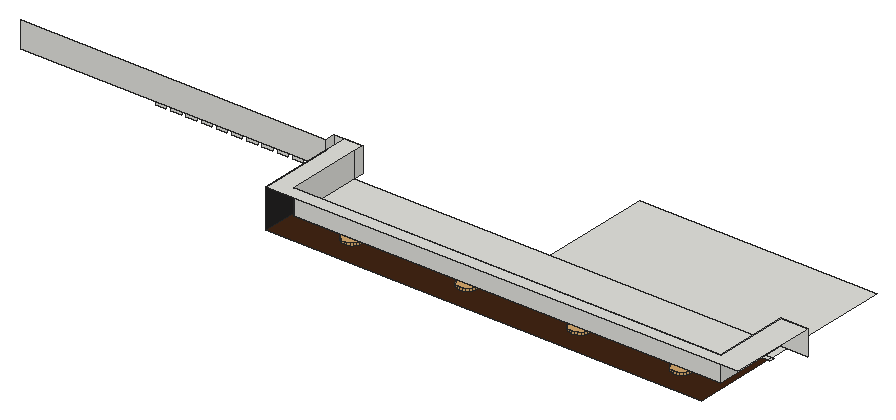
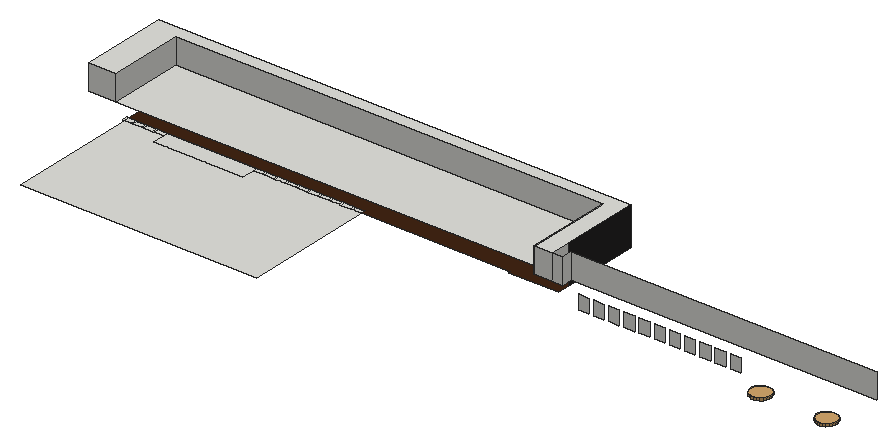
# SketchUp Ruby script. Lengths in inches.
U = 1.inch
M = Sketchup.active_model
def pt(a) = Geom::Point3d.new(a.map { |v| v * U })
def face(e, loops, mat)
  f = e.add_face(loops[0].map { |a| pt(a) })
  loops[1..].each { |l| e.add_face(l.map { |a| pt(a) }).erase! }
  f.material = f.back_material = mat if mat
  f
end
# faces: each face lists its corners as indices into pts; further lists are holes
def faces(e, pts, list, mat = nil) = list.each { |f| face(e, (f[0].is_a?(Array) ? f : [f]).map { |l| l.map { |i| pts[i] } }, mat) }
# xy, xz, yz: faces in a plane at the given z, y or x. An outline is a flat list of corners, or four numbers for a rectangle; further outlines are holes
def ring(l) = l.size == 4 ? [[l[0], l[1]], [l[2], l[1]], [l[2], l[3]], [l[0], l[3]]] : l.each_slice(2).to_a
def flat(e, list, mat, &to3) = list.each { |f| face(e, (f[0].is_a?(Array) ? f : [f]).map { |l| ring(l).map { |u, v| to3.(u, v) } }, mat) }
def xy(e, z, list, mat = nil) = flat(e, list, mat) { |x, y| [x, y, z] }
def xz(e, y, list, mat = nil) = flat(e, list, mat) { |x, z| [x, y, z] }
def yz(e, x, list, mat = nil) = flat(e, list, mat) { |y, z| [x, y, z] }
def lines(e, pts, list) = list.each { |a, b| e.add_line(pt(pts[a]), pt(pts[b])) }
# prism: a flat outline (further loops are holes) pulled along v
def prism(e, loops, v, mat = nil)
  f = face(e, loops, mat); d = Geom::Vector3d.new(v.map { |x| x * U })
  f.pushpull(f.normal.samedirection?(d) ? d.length : -d.length)
end
def box(e, o, s, mat = nil) = prism(e, [[o, [o[0] + s[0], o[1], o[2]], [o[0] + s[0], o[1] + s[1], o[2]], [o[0], o[1] + s[1], o[2]]]], [0, 0, s[2]], mat)
def at(x, y, z, deg = 0) = Geom::Transformation.translation(pt([x, y, z])) * Geom::Transformation.rotation(ORIGIN, Z_AXIS, deg.degrees)
def axes(o, x, y, z) = Geom::Transformation.new([*x, 0, *y, 0, *z, 0, *pt(o).to_a, 1])
def part(name) = M.definitions.add(name)
# library, detail: a bought-in or finely detailed component or shape, given as its bounding box
def library(name, o, s) = part(name).tap { |d| box(d.entities, o, s) }
def detail(e, o, s) = box(e.add_group.entities, o, s)
def put(e, d, t, mat = nil) = e.add_instance(d, t).tap { |i| i.material = mat if mat }
def group(e, t, mat = nil) = e.add_group.tap { |g| g.transformation = t; g.material = mat if mat }.entities
root = M.entities
M.materials.add("[Field Square Tile]").color = [211, 167, 108]
M.materials.add("[Granite Dark Gray]").color = [38, 37, 37]
M.materials.add("[Wood Veneer 01]").color = [66, 38, 20]
xy(root,380.5,[[534.46,2343.96,539.88,2346.71],[539.88,2343.96,541.08,2346.71],[541.08,2343.96,546.51,2346.71],[546.51,2343.96,547.71,2346.71],[547.71,2343.96,553.13,2346.71],
  [553.13,2343.96,554.33,2346.71],[554.33,2343.96,559.76,2346.71],[559.76,2343.96,560.96,2346.71],[560.96,2343.96,566.38,2346.71],[566.38,2343.96,567.58,2346.71],
  [567.58,2343.96,573.01,2346.71],[573.01,2343.96,574.21,2346.71],[574.21,2343.96,579.63,2346.71],[579.63,2343.96,580.83,2346.71],[580.83,2343.96,586.26,2346.71],
  [586.26,2343.96,587.46,2346.71],[587.46,2343.96,592.88,2346.71],[592.88,2343.96,594.08,2346.71],[594.08,2343.96,599.51,2346.71],[599.51,2343.96,653.06,2354.27],
  [653.06,2343.96,658.48,2346.71],[658.48,2343.96,659.68,2346.71],[659.68,2343.96,665.11,2346.71],[665.11,2343.96,666.31,2346.71],[666.31,2343.96,671.73,2346.71],
  [671.73,2343.96,672.56,2346.71],[672.56,2343.96,676.54,2346.71],[676.54,2343.96,677.98,2346.71],[534.46,2346.71,534.46,2425.46,676.54,2425.46,676.54,2346.71,653.06,2346.71,653.06,2354.27,599.51,2354.27,599.51,2346.71]])
xy(root,380.5,[[[414.98,2294.125,414.98,2347.9,444.78,2347.9,444.78,2346.71,534.46,2346.71,534.46,2343.96,676.54,2343.96,676.54,2294.125],[521.68,2306.32,523.23,2306.53,524.68,2307.13,525.92,2308.08,526.88,2309.32,527.48,2310.77,527.68,2312.32,527.48,2313.88,526.88,2315.32,525.92,2316.57,524.68,2317.52,523.23,2318.12,521.68,2318.32,520.13,2318.12,518.68,2317.52,517.4375,2316.57,516.49,2315.32,515.89,2313.88,515.68,2312.32,515.89,2310.77,516.49,2309.32,517.4375,2308.08,518.68,2307.13,520.13,2306.53],[588.96,2306.32,590.51,2306.53,591.96,2307.13,593.2,2308.08,594.16,2309.32,594.76,2310.77,594.96,2312.32,594.76,2313.88,594.16,2315.32,593.2,2316.57,591.96,2317.52,590.51,2318.12,588.96,2318.32,587.41,2318.12,585.96,2317.52,584.72,2316.57,583.76,2315.32,583.16,2313.88,582.96,2312.32,583.16,2310.77,583.76,2309.32,584.72,2308.08,585.96,2307.13,587.41,2306.53],[650.33,2306.32,651.89,2306.53,653.33,2307.13,654.58,2308.08,655.53,2309.32,656.13,2310.77,656.33,2312.32,656.13,2313.88,655.53,2315.32,654.58,2316.57,653.33,2317.52,651.89,2318.12,650.33,2318.32,648.78,2318.12,647.33,2317.52,646.09,2316.57,645.14,2315.32,644.54,2313.88,644.33,2312.32,644.54,2310.77,645.14,2309.32,646.09,2308.08,647.33,2307.13,648.78,2306.53],[452.22,2306.32,453.77,2306.53,455.22,2307.13,456.46,2308.08,457.41,2309.32,458.01,2310.77,458.22,2312.32,458.01,2313.88,457.41,2315.32,456.46,2316.57,455.22,2317.52,453.77,2318.12,452.22,2318.32,450.67,2318.12,449.22,2317.52,447.98,2316.57,447.02,2315.32,446.42,2313.88,446.22,2312.32,446.42,2310.77,447.02,2309.32,447.98,2308.08,449.22,2307.13,450.67,2306.53]]],"[Wood Veneer 01]")
xy(root,381.8125,[[452.22,2306.32,450.67,2306.53,449.22,2307.13,447.98,2308.08,447.02,2309.32,446.42,2310.77,446.22,2312.32,446.42,2313.88,447.02,2315.32,447.98,2316.57,449.22,2317.52,450.67,2318.12,452.22,2318.32,453.77,2318.12,455.22,2317.52,456.46,2316.57,457.41,2315.32,458.01,2313.88,458.22,2312.32,458.01,2310.77,457.41,2309.32,456.46,2308.08,455.22,2307.13,453.77,2306.53],[521.68,2306.32,520.13,2306.53,518.68,2307.13,517.4375,2308.08,516.49,2309.32,515.89,2310.77,515.68,2312.32,515.89,2313.88,516.49,2315.32,517.4375,2316.57,518.68,2317.52,520.13,2318.12,521.68,2318.32,523.23,2318.12,524.68,2317.52,525.92,2316.57,526.88,2315.32,527.48,2313.88,527.68,2312.32,527.48,2310.77,526.88,2309.32,525.92,2308.08,524.68,2307.13,523.23,2306.53],[588.96,2306.32,587.41,2306.53,585.96,2307.13,584.72,2308.08,583.76,2309.32,583.16,2310.77,582.96,2312.32,583.16,2313.88,583.76,2315.32,584.72,2316.57,585.96,2317.52,587.41,2318.12,588.96,2318.32,590.51,2318.12,591.96,2317.52,593.2,2316.57,594.16,2315.32,594.76,2313.88,594.96,2312.32,594.76,2310.77,594.16,2309.32,593.2,2308.08,591.96,2307.13,590.51,2306.53],[650.33,2306.32,648.78,2306.53,647.33,2307.13,646.09,2308.08,645.14,2309.32,644.54,2310.77,644.33,2312.32,644.54,2313.88,645.14,2315.32,646.09,2316.57,647.33,2317.52,648.78,2318.12,650.33,2318.32,651.89,2318.12,653.33,2317.52,654.58,2316.57,655.53,2315.32,656.13,2313.88,656.33,2312.32,656.13,2310.77,655.53,2309.32,654.58,2308.08,653.33,2307.13,651.89,2306.53]],"[Field Square Tile]")
xy(root,381.875,[[240.83,2359.13,239.27,2359.16,237.76,2359.6,236.42,2360.41,235.34,2361.54,234.58,2362.91,234.21,2364.4375,234.24,2366,234.68,2367.51,235.49,2368.85,236.62,2369.93,237.99,2370.69,239.51,2371.06,241.08,2371.03,242.58,2370.59,243.92,2369.78,245.01,2368.65,245.76,2367.28,246.14,2365.75,246.1,2364.1875,245.67,2362.68,244.86,2361.34,243.73,2360.26,242.35,2359.51],[280.58,2359.13,279.02,2359.16,277.51,2359.6,276.17,2360.41,275.09,2361.54,274.33,2362.91,273.96,2364.4375,273.99,2366,274.43,2367.51,275.24,2368.85,276.37,2369.93,277.74,2370.69,279.26,2371.06,280.83,2371.03,282.33,2370.59,283.67,2369.78,284.76,2368.65,285.51,2367.28,285.89,2365.75,285.85,2364.1875,285.42,2362.68,284.61,2361.34,283.48,2360.26,282.1,2359.51]],"[Field Square Tile]")
xy(root,388.625,[[425.6875,2301.68,682.18,2346.71]])
xy(root,403.8125,[[414.98,2294.125,698.16,2294.125,698.16,2346.71,682.18,2346.71,682.18,2301.68,425.6875,2301.68,425.6875,2353.05,414.98,2353.05]])
xz(root,2301.68,[[425.6875,388.625,682.18,403.8125]])
xz(root,2346.49,[[225.31,388.625,408.63,403.8125]])
xz(root,2346.71,[[682.18,388.625,698.16,403.8125]])
xz(root,2353.05,[[408.63,388.625,414.98,403.8125],[414.98,388.625,425.6875,403.8125]])
xz(root,2355.06,[[299.93,380.5,306.18,388.625],[309.06,380.5,315.31,388.625],[318.18,380.5,324.43,388.625],[327.31,380.5,333.56,388.625],[336.43,380.5,342.68,388.625],
  [345.56,380.5,351.81,388.625],[354.68,380.5,360.93,388.625],[363.81,380.5,370.06,388.625],[372.93,380.5,379.18,388.625],[382.06,380.5,388.31,388.625],
  [391.18,380.5,397.43,388.625]])
yz(root,408.63,[[2346.49,388.625,2353.05,403.8125]])
yz(root,414.98,[[2294.125,380.5,2340.15,403.8125]],"[Granite Dark Gray]")
yz(root,425.6875,[[2301.68,388.625,2346.71,403.8125],[2346.71,388.625,2353.05,403.8125]])
yz(root,682.18,[[2301.68,388.625,2346.71,403.8125]])
p = [[452.22,2306.32,380.5],[450.67,2306.53,380.5],[450.67,2306.53,381.8125],[452.22,2306.32,381.8125],[453.77,2306.53,380.5],[453.77,2306.53,381.8125],
  [521.68,2306.32,380.5],[520.13,2306.53,380.5],[520.13,2306.53,381.8125],[521.68,2306.32,381.8125],[523.23,2306.53,380.5],[523.23,2306.53,381.8125],
  [588.96,2306.32,380.5],[587.41,2306.53,380.5],[587.41,2306.53,381.8125],[588.96,2306.32,381.8125],[590.51,2306.53,380.5],[590.51,2306.53,381.8125],
  [650.33,2306.32,380.5],[648.78,2306.53,380.5],[648.78,2306.53,381.8125],[650.33,2306.32,381.8125],[651.89,2306.53,380.5],[651.89,2306.53,381.8125],
  [449.22,2307.13,380.5],[449.22,2307.13,381.8125],[455.22,2307.13,380.5],[455.22,2307.13,381.8125],[518.68,2307.13,380.5],[518.68,2307.13,381.8125],
  [524.68,2307.13,380.5],[524.68,2307.13,381.8125],[585.96,2307.13,380.5],[585.96,2307.13,381.8125],[591.96,2307.13,380.5],[591.96,2307.13,381.8125],
  [647.33,2307.13,380.5],[647.33,2307.13,381.8125],[653.33,2307.13,380.5],[653.33,2307.13,381.8125],[447.98,2308.08,380.5],[447.98,2308.08,381.8125],
  [456.46,2308.08,380.5],[456.46,2308.08,381.8125],[517.4375,2308.08,380.5],[517.4375,2308.08,381.8125],[525.92,2308.08,380.5],[525.92,2308.08,381.8125],
  [584.72,2308.08,380.5],[584.72,2308.08,381.8125],[593.2,2308.08,380.5],[593.2,2308.08,381.8125],[646.09,2308.08,380.5],[646.09,2308.08,381.8125],
  [654.58,2308.08,380.5],[654.58,2308.08,381.8125],[447.02,2309.32,380.5],[447.02,2309.32,381.8125],[457.41,2309.32,380.5],[457.41,2309.32,381.8125],
  [516.49,2309.32,380.5],[516.49,2309.32,381.8125],[526.88,2309.32,380.5],[526.88,2309.32,381.8125],[583.76,2309.32,380.5],[583.76,2309.32,381.8125],
  [594.16,2309.32,380.5],[594.16,2309.32,381.8125],[645.14,2309.32,380.5],[645.14,2309.32,381.8125],[655.53,2309.32,380.5],[655.53,2309.32,381.8125],
  [446.42,2310.77,380.5],[446.42,2310.77,381.8125],[458.01,2310.77,380.5],[458.01,2310.77,381.8125],[515.89,2310.77,380.5],[515.89,2310.77,381.8125],
  [527.48,2310.77,380.5],[527.48,2310.77,381.8125],[583.16,2310.77,380.5],[583.16,2310.77,381.8125],[594.76,2310.77,380.5],[594.76,2310.77,381.8125],
  [644.54,2310.77,380.5],[644.54,2310.77,381.8125],[656.13,2310.77,380.5],[656.13,2310.77,381.8125],[446.22,2312.32,380.5],[446.22,2312.32,381.8125],
  [458.22,2312.32,380.5],[458.22,2312.32,381.8125],[515.68,2312.32,380.5],[515.68,2312.32,381.8125],[527.68,2312.32,380.5],[527.68,2312.32,381.8125],
  [582.96,2312.32,380.5],[582.96,2312.32,381.8125],[594.96,2312.32,380.5],[594.96,2312.32,381.8125],[644.33,2312.32,380.5],[644.33,2312.32,381.8125],
  [656.33,2312.32,380.5],[656.33,2312.32,381.8125],[446.42,2313.88,380.5],[446.42,2313.88,381.8125],[458.01,2313.88,380.5],[458.01,2313.88,381.8125],
  [515.89,2313.88,380.5],[515.89,2313.88,381.8125],[527.48,2313.88,380.5],[527.48,2313.88,381.8125],[583.16,2313.88,380.5],[583.16,2313.88,381.8125],
  [594.76,2313.88,380.5],[594.76,2313.88,381.8125],[644.54,2313.88,380.5],[644.54,2313.88,381.8125],[656.13,2313.88,380.5],[656.13,2313.88,381.8125],
  [447.02,2315.32,380.5],[447.02,2315.32,381.8125],[457.41,2315.32,380.5],[457.41,2315.32,381.8125],[516.49,2315.32,380.5],[516.49,2315.32,381.8125],
  [526.88,2315.32,380.5],[526.88,2315.32,381.8125],[583.76,2315.32,380.5],[583.76,2315.32,381.8125],[594.16,2315.32,380.5],[594.16,2315.32,381.8125],
  [645.14,2315.32,380.5],[645.14,2315.32,381.8125],[655.53,2315.32,380.5],[655.53,2315.32,381.8125],[447.98,2316.57,380.5],[447.98,2316.57,381.8125],
  [456.46,2316.57,380.5],[456.46,2316.57,381.8125],[517.4375,2316.57,380.5],[517.4375,2316.57,381.8125],[525.92,2316.57,380.5],[525.92,2316.57,381.8125],
  [584.72,2316.57,380.5],[584.72,2316.57,381.8125],[593.2,2316.57,380.5],[593.2,2316.57,381.8125],[646.09,2316.57,380.5],[646.09,2316.57,381.8125],
  [654.58,2316.57,380.5],[654.58,2316.57,381.8125],[449.22,2317.52,380.5],[449.22,2317.52,381.8125],[455.22,2317.52,380.5],[455.22,2317.52,381.8125],
  [518.68,2317.52,380.5],[518.68,2317.52,381.8125],[524.68,2317.52,380.5],[524.68,2317.52,381.8125],[585.96,2317.52,380.5],[585.96,2317.52,381.8125],
  [591.96,2317.52,380.5],[591.96,2317.52,381.8125],[647.33,2317.52,380.5],[647.33,2317.52,381.8125],[653.33,2317.52,380.5],[653.33,2317.52,381.8125],
  [450.67,2318.12,380.5],[450.67,2318.12,381.8125],[453.77,2318.12,380.5],[453.77,2318.12,381.8125],[520.13,2318.12,380.5],[520.13,2318.12,381.8125],
  [523.23,2318.12,380.5],[523.23,2318.12,381.8125],[587.41,2318.12,380.5],[587.41,2318.12,381.8125],[590.51,2318.12,380.5],[590.51,2318.12,381.8125],
  [648.78,2318.12,380.5],[648.78,2318.12,381.8125],[651.89,2318.12,380.5],[651.89,2318.12,381.8125],[452.22,2318.32,380.5],[452.22,2318.32,381.8125],
  [521.68,2318.32,380.5],[521.68,2318.32,381.8125],[588.96,2318.32,380.5],[588.96,2318.32,381.8125],[650.33,2318.32,380.5],[650.33,2318.32,381.8125],
  [240.83,2359.13,380.5],[239.27,2359.16,380.5],[239.27,2359.16,381.875],[240.83,2359.13,381.875],[242.35,2359.51,380.5],[242.35,2359.51,381.875],
  [280.58,2359.13,380.5],[279.02,2359.16,380.5],[279.02,2359.16,381.875],[280.58,2359.13,381.875],[282.1,2359.51,380.5],[282.1,2359.51,381.875],
  [237.76,2359.6,380.5],[237.76,2359.6,381.875],[277.51,2359.6,380.5],[277.51,2359.6,381.875],[243.73,2360.26,380.5],[243.73,2360.26,381.875],
  [283.48,2360.26,380.5],[283.48,2360.26,381.875],[236.42,2360.41,380.5],[236.42,2360.41,381.875],[276.17,2360.41,380.5],[276.17,2360.41,381.875],
  [244.86,2361.34,380.5],[244.86,2361.34,381.875],[284.61,2361.34,380.5],[284.61,2361.34,381.875],[235.34,2361.54,380.5],[235.34,2361.54,381.875],
  [275.09,2361.54,380.5],[275.09,2361.54,381.875],[245.67,2362.68,380.5],[245.67,2362.68,381.875],[285.42,2362.68,380.5],[285.42,2362.68,381.875],
  [234.58,2362.91,380.5],[234.58,2362.91,381.875],[274.33,2362.91,380.5],[274.33,2362.91,381.875],[246.1,2364.1875,380.5],[246.1,2364.1875,381.875],
  [285.85,2364.1875,380.5],[285.85,2364.1875,381.875],[234.21,2364.4375,380.5],[234.21,2364.4375,381.875],[273.96,2364.4375,380.5],[273.96,2364.4375,381.875],
  [246.14,2365.75,380.5],[246.14,2365.75,381.875],[285.89,2365.75,380.5],[285.89,2365.75,381.875],[234.24,2366,380.5],[234.24,2366,381.875],
  [273.99,2366,380.5],[273.99,2366,381.875],[245.76,2367.28,380.5],[245.76,2367.28,381.875],[285.51,2367.28,380.5],[285.51,2367.28,381.875],
  [234.68,2367.51,380.5],[234.68,2367.51,381.875],[274.43,2367.51,380.5],[274.43,2367.51,381.875],[245.01,2368.65,380.5],[245.01,2368.65,381.875],
  [284.76,2368.65,380.5],[284.76,2368.65,381.875],[235.49,2368.85,380.5],[235.49,2368.85,381.875],[275.24,2368.85,380.5],[275.24,2368.85,381.875],
  [243.92,2369.78,380.5],[243.92,2369.78,381.875],[283.67,2369.78,380.5],[283.67,2369.78,381.875],[236.62,2369.93,380.5],[236.62,2369.93,381.875],
  [276.37,2369.93,380.5],[276.37,2369.93,381.875],[242.58,2370.59,380.5],[242.58,2370.59,381.875],[282.33,2370.59,380.5],[282.33,2370.59,381.875],
  [237.99,2370.69,380.5],[237.99,2370.69,381.875],[277.74,2370.69,380.5],[277.74,2370.69,381.875],[241.08,2371.03,380.5],[241.08,2371.03,381.875],
  [280.83,2371.03,380.5],[280.83,2371.03,381.875],[239.51,2371.06,380.5],[239.51,2371.06,381.875],[279.26,2371.06,380.5],[279.26,2371.06,381.875],
  [415,2303.93,380.5],[414.98,2294.125,380.5]]
faces(root,p,[[0,1,2,3],[4,0,3,5],[6,7,8,9],[10,6,9,11],[12,13,14,15],[16,12,15,17],[18,19,20,21],[22,18,21,23],
  [1,24,25,2],[26,4,5,27],[7,28,29,8],[30,10,11,31],[13,32,33,14],[34,16,17,35],[19,36,37,20],[38,22,23,39],
  [24,40,41,25],[42,26,27,43],[28,44,45,29],[46,30,31,47],[32,48,49,33],[50,34,35,51],[36,52,53,37],[54,38,39,55],
  [40,56,57,41],[58,42,43,59],[44,60,61,45],[62,46,47,63],[48,64,65,49],[66,50,51,67],[52,68,69,53],[70,54,55,71],
  [56,72,73,57],[74,58,59,75],[60,76,77,61],[78,62,63,79],[64,80,81,65],[82,66,67,83],[68,84,85,69],[86,70,71,87],
  [72,88,89,73],[90,74,75,91],[76,92,93,77],[94,78,79,95],[80,96,97,81],[98,82,83,99],[84,100,101,85],[102,86,87,103],
  [88,104,105,89],[106,90,91,107],[92,108,109,93],[110,94,95,111],[96,112,113,97],[114,98,99,115],[100,116,117,101],[118,102,103,119],
  [104,120,121,105],[122,106,107,123],[108,124,125,109],[126,110,111,127],[112,128,129,113],[130,114,115,131],[116,132,133,117],[134,118,119,135],
  [120,136,137,121],[138,122,123,139],[124,140,141,125],[142,126,127,143],[128,144,145,129],[146,130,131,147],[132,148,149,133],[150,134,135,151],
  [136,152,153,137],[154,138,139,155],[140,156,157,141],[158,142,143,159],[144,160,161,145],[162,146,147,163],[148,164,165,149],[166,150,151,167],
  [152,168,169,153],[170,154,155,171],[156,172,173,157],[174,158,159,175],[160,176,177,161],[178,162,163,179],[164,180,181,165],[182,166,167,183],
  [168,184,185,169],[184,170,171,185],[172,186,187,173],[186,174,175,187],[176,188,189,177],[188,178,179,189],[180,190,191,181],[190,182,183,191],
  [192,193,194,195],[196,192,195,197],[198,199,200,201],[202,198,201,203],[193,204,205,194],[199,206,207,200],[208,196,197,209],[210,202,203,211],
  [204,212,213,205],[206,214,215,207],[216,208,209,217],[218,210,211,219],[212,220,221,213],[214,222,223,215],[224,216,217,225],[226,218,219,227],
  [220,228,229,221],[222,230,231,223],[232,224,225,233],[234,226,227,235],[228,236,237,229],[230,238,239,231],[240,232,233,241],[242,234,235,243],
  [236,244,245,237],[238,246,247,239],[248,240,241,249],[250,242,243,251],[244,252,253,245],[246,254,255,247],[256,248,249,257],[258,250,251,259],
  [252,260,261,253],[254,262,263,255],[264,256,257,265],[266,258,259,267],[260,268,269,261],[262,270,271,263],[272,264,265,273],[274,266,267,275],
  [268,276,277,269],[270,278,279,271],[280,272,273,281],[282,274,275,283],[276,284,285,277],[278,286,287,279],[284,280,281,285],[286,282,283,287]],"[Field Square Tile]")
lines(root,p,[[288,289]])
